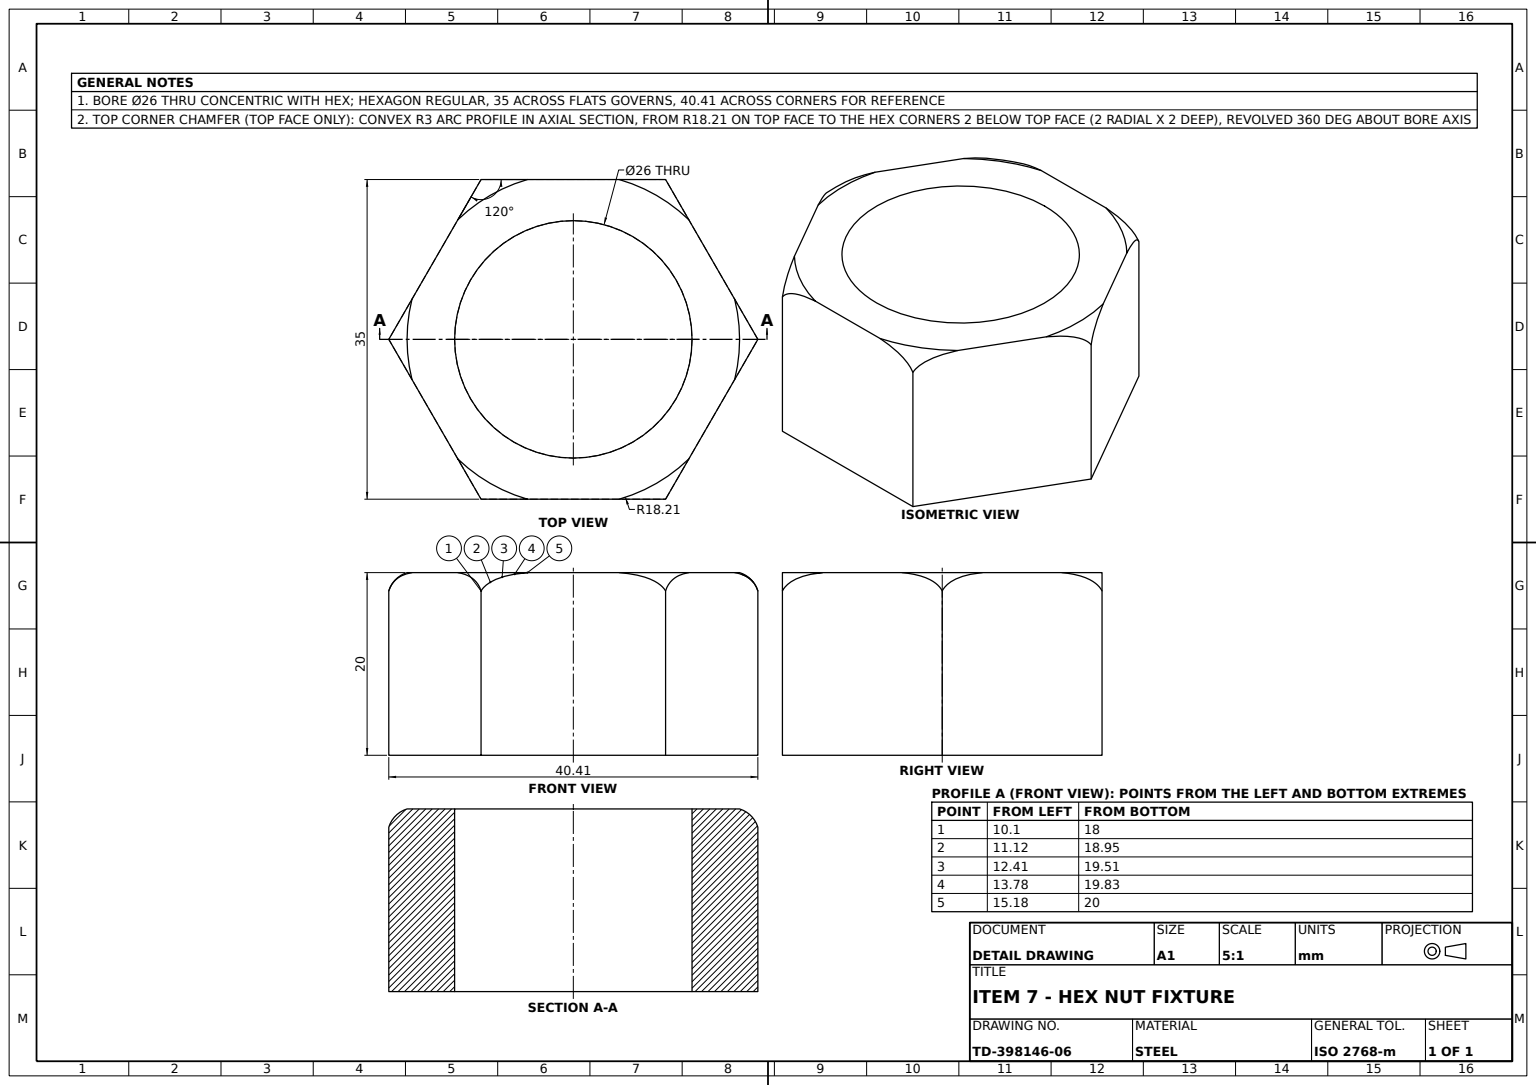
ISO-10303-21;
HEADER;
FILE_DESCRIPTION((''),'2;1');
FILE_NAME('','',(''),(''),'','','');
FILE_SCHEMA(('AUTOMOTIVE_DESIGN'));
ENDSEC;
DATA;
#1=APPLICATION_CONTEXT('');
#2=PRODUCT_CONTEXT('',#1,'mechanical');
#3=PRODUCT('','','',(#2));
#4=PRODUCT_DEFINITION_FORMATION('','',#3);
#5=PRODUCT_DEFINITION_CONTEXT('',#1,'design');
#6=PRODUCT_DEFINITION('','',#4,#5);
#7=PRODUCT_DEFINITION_SHAPE('','',#6);
#8=(LENGTH_UNIT()NAMED_UNIT(*)SI_UNIT(.MILLI.,.METRE.));
#9=(NAMED_UNIT(*)PLANE_ANGLE_UNIT()SI_UNIT($,.RADIAN.));
#10=(NAMED_UNIT(*)SI_UNIT($,.STERADIAN.)SOLID_ANGLE_UNIT());
#11=UNCERTAINTY_MEASURE_WITH_UNIT(LENGTH_MEASURE(1.E-05),#8,'distance_accuracy_value','');
#12=(GEOMETRIC_REPRESENTATION_CONTEXT(3)GLOBAL_UNCERTAINTY_ASSIGNED_CONTEXT((#11))GLOBAL_UNIT_ASSIGNED_CONTEXT((#8,#9,#10))REPRESENTATION_CONTEXT('',''));
#13=CARTESIAN_POINT('',(-10.10363,8.,17.5));
#14=VERTEX_POINT('',#13);
#15=CARTESIAN_POINT('',(-12.642762,10.,13.102094));
#16=VERTEX_POINT('',#15);
#17=CARTESIAN_POINT('',(-10.165722,8.204696,17.392454));
#18=CARTESIAN_POINT('',(-10.243014,8.380727,17.258579));
#19=CARTESIAN_POINT('',(-10.416921,8.69635,16.957363));
#20=CARTESIAN_POINT('',(-10.51443,8.835748,16.788473));
#21=CARTESIAN_POINT('',(-10.715898,9.077372,16.43952));
#22=CARTESIAN_POINT('',(-10.820898,9.181438,16.257655));
#23=CARTESIAN_POINT('',(-11.03705,9.365421,15.883269));
#24=CARTESIAN_POINT('',(-11.148709,9.445473,15.68987));
#25=CARTESIAN_POINT('',(-11.485835,9.654439,15.105951));
#26=CARTESIAN_POINT('',(-11.714336,9.754069,14.710176));
#27=CARTESIAN_POINT('',(-12.175668,9.907509,13.911124));
#28=CARTESIAN_POINT('',(-12.408551,9.960782,13.507759));
#29=B_SPLINE_CURVE_WITH_KNOTS('',3,(#13,#17,#18,#19,#20,#21,#22,#23,#24,#25,#26,#27,#28,#15),.UNSPECIFIED.,.F.,.F.,(4,2,2,2,2,2,4),(0.000000229,0.000702604,0.001404979,0.002107355,0.00280973,0.004214481,0.005619231),.UNSPECIFIED.);
#30=EDGE_CURVE('',#14,#16,#29,.T.);
#31=ORIENTED_EDGE('',*,*,#30,.F.);
#32=CARTESIAN_POINT('',(-5.025365,10.,17.5));
#33=VERTEX_POINT('',#32);
#34=CARTESIAN_POINT('',(-5.492104,9.960923,17.5));
#35=CARTESIAN_POINT('',(-5.960143,9.907453,17.5));
#36=CARTESIAN_POINT('',(-6.884053,9.753721,17.5));
#37=CARTESIAN_POINT('',(-7.33942,9.654067,17.5));
#38=CARTESIAN_POINT('',(-8.006087,9.447914,17.5));
#39=CARTESIAN_POINT('',(-8.225551,9.369653,17.5));
#40=CARTESIAN_POINT('',(-8.65696,9.187123,17.5));
#41=CARTESIAN_POINT('',(-8.870751,9.081899,17.5));
#42=CARTESIAN_POINT('',(-9.277733,8.838784,17.5));
#43=CARTESIAN_POINT('',(-9.470105,8.701958,17.5));
#44=CARTESIAN_POINT('',(-9.822347,8.383681,17.5));
#45=CARTESIAN_POINT('',(-9.980357,8.203194,17.5));
#46=B_SPLINE_CURVE_WITH_KNOTS('',3,(#32,#34,#35,#36,#37,#38,#39,#40,#41,#42,#43,#44,#45,#13),.UNSPECIFIED.,.F.,.F.,(4,2,2,2,2,2,4),(0.00502645,0.006430133,0.007833817,0.008535659,0.009237501,0.009939343,0.010641184),.UNSPECIFIED.);
#47=EDGE_CURVE('',#33,#14,#46,.T.);
#48=ORIENTED_EDGE('',*,*,#47,.F.);
#49=CARTESIAN_POINT('',(0.,10.,0.));
#50=DIRECTION('',(0.,-1.,0.));
#51=DIRECTION('',(0.,0.,-1.));
#52=AXIS2_PLACEMENT_3D('',#49,#50,#51);
#53=CIRCLE('',#52,18.207259);
#54=EDGE_CURVE('',#33,#16,#53,.T.);
#55=ORIENTED_EDGE('',*,*,#54,.T.);
#56=EDGE_LOOP('',(#31,#48,#55));
#57=FACE_OUTER_BOUND('',#56,.T.);
#58=CARTESIAN_POINT('',(0.,7.129171,0.));
#59=AXIS2_PLACEMENT_3D('',#58,#50,#51);
#60=TOROIDAL_SURFACE('',#59,17.336431,3.);
#61=ADVANCED_FACE('',(#57),#60,.T.);
#62=CARTESIAN_POINT('',(-10.10363,-10.,17.5));
#63=VERTEX_POINT('',#62);
#64=CARTESIAN_POINT('',(-10.10363,10.,17.5));
#65=VECTOR('',#50,1000.);
#66=LINE('',#64,#65);
#67=EDGE_CURVE('',#14,#63,#66,.T.);
#68=ORIENTED_EDGE('',*,*,#67,.F.);
#69=ORIENTED_EDGE('',*,*,#30,.T.);
#70=CARTESIAN_POINT('',(-17.668127,10.,4.397906));
#71=VERTEX_POINT('',#70);
#72=CARTESIAN_POINT('',(-20.207259,10.,0.));
#73=DIRECTION('',(0.5,0.,0.866025404));
#74=VECTOR('',#73,1000.);
#75=LINE('',#72,#74);
#76=EDGE_CURVE('',#71,#16,#75,.T.);
#77=ORIENTED_EDGE('',*,*,#76,.F.);
#78=CARTESIAN_POINT('',(-20.207259,8.,0.));
#79=VERTEX_POINT('',#78);
#80=CARTESIAN_POINT('',(-17.902082,9.960825,3.992684));
#81=CARTESIAN_POINT('',(-18.134693,9.907626,3.58979));
#82=CARTESIAN_POINT('',(-18.595438,9.754498,2.791757));
#83=CARTESIAN_POINT('',(-18.823622,9.655098,2.396531));
#84=CARTESIAN_POINT('',(-19.160225,9.446798,1.813516));
#85=CARTESIAN_POINT('',(-19.271845,9.366951,1.620186));
#86=CARTESIAN_POINT('',(-19.488371,9.182983,1.245151));
#87=CARTESIAN_POINT('',(-19.593676,9.078818,1.062757));
#88=CARTESIAN_POINT('',(-19.796013,8.836412,0.7123));
#89=CARTESIAN_POINT('',(-19.892647,8.698371,0.544925));
#90=CARTESIAN_POINT('',(-20.066575,8.383458,0.243673));
#91=CARTESIAN_POINT('',(-20.145542,8.203461,0.106897));
#92=B_SPLINE_CURVE_WITH_KNOTS('',3,(#70,#80,#81,#82,#83,#84,#85,#86,#87,#88,#89,#90,#91,#78),.UNSPECIFIED.,.F.,.F.,(4,2,2,2,2,2,4),(0.000002385,0.001403147,0.002803908,0.003504289,0.004204669,0.00490505,0.005605431),.UNSPECIFIED.);
#93=EDGE_CURVE('',#71,#79,#92,.T.);
#94=ORIENTED_EDGE('',*,*,#93,.T.);
#95=CARTESIAN_POINT('',(-20.207259,-10.,0.));
#96=VERTEX_POINT('',#95);
#97=LINE('',#72,#65);
#98=EDGE_CURVE('',#79,#96,#97,.T.);
#99=ORIENTED_EDGE('',*,*,#98,.T.);
#100=LINE('',#95,#74);
#101=EDGE_CURVE('',#96,#63,#100,.T.);
#102=ORIENTED_EDGE('',*,*,#101,.T.);
#103=EDGE_LOOP('',(#68,#69,#77,#94,#99,#102));
#104=FACE_OUTER_BOUND('',#103,.T.);
#105=DIRECTION('',(0.866025404,0.,-0.5));
#106=DIRECTION('',(-0.5,0.,-0.866025404));
#107=AXIS2_PLACEMENT_3D('',#72,#105,#106);
#108=PLANE('',#107);
#109=ADVANCED_FACE('',(#104),#108,.F.);
#110=CARTESIAN_POINT('',(10.10363,8.,-17.5));
#111=VERTEX_POINT('',#110);
#112=CARTESIAN_POINT('',(10.10363,-10.,-17.5));
#113=VERTEX_POINT('',#112);
#114=CARTESIAN_POINT('',(10.10363,10.,-17.5));
#115=LINE('',#114,#65);
#116=EDGE_CURVE('',#111,#113,#115,.T.);
#117=ORIENTED_EDGE('',*,*,#116,.T.);
#118=CARTESIAN_POINT('',(-10.10363,-10.,-17.5));
#119=VERTEX_POINT('',#118);
#120=DIRECTION('',(-1.,0.,0.));
#121=VECTOR('',#120,1000.);
#122=LINE('',#112,#121);
#123=EDGE_CURVE('',#113,#119,#122,.T.);
#124=ORIENTED_EDGE('',*,*,#123,.T.);
#125=CARTESIAN_POINT('',(-10.10363,8.,-17.5));
#126=VERTEX_POINT('',#125);
#127=CARTESIAN_POINT('',(-10.10363,10.,-17.5));
#128=LINE('',#127,#65);
#129=EDGE_CURVE('',#126,#119,#128,.T.);
#130=ORIENTED_EDGE('',*,*,#129,.F.);
#131=CARTESIAN_POINT('',(-5.025365,10.,-17.5));
#132=VERTEX_POINT('',#131);
#133=CARTESIAN_POINT('',(-9.98061,8.202777,-17.5));
#134=CARTESIAN_POINT('',(-9.825141,8.380727,-17.5));
#135=CARTESIAN_POINT('',(-9.473221,8.699564,-17.5));
#136=CARTESIAN_POINT('',(-9.282037,8.835729,-17.5));
#137=CARTESIAN_POINT('',(-8.87945,9.077171,-17.5));
#138=CARTESIAN_POINT('',(-8.666501,9.182682,-17.5));
#139=CARTESIAN_POINT('',(-8.233223,9.366796,-17.5));
#140=CARTESIAN_POINT('',(-8.012779,9.445661,-17.5));
#141=CARTESIAN_POINT('',(-7.343094,9.653291,-17.5));
#142=CARTESIAN_POINT('',(-6.885612,9.753482,-17.5));
#143=CARTESIAN_POINT('',(-5.957388,9.90789,-17.5));
#144=CARTESIAN_POINT('',(-5.491532,9.960971,-17.5));
#145=B_SPLINE_CURVE_WITH_KNOTS('',3,(#125,#133,#134,#135,#136,#137,#138,#139,#140,#141,#142,#143,#144,#131),.UNSPECIFIED.,.F.,.F.,(4,2,2,2,2,2,4),(0.035514707,0.036213744,0.036912782,0.037611819,0.038310856,0.039708931,0.041107005),.UNSPECIFIED.);
#146=EDGE_CURVE('',#126,#132,#145,.T.);
#147=ORIENTED_EDGE('',*,*,#146,.T.);
#148=CARTESIAN_POINT('',(5.025365,10.,-17.5));
#149=VERTEX_POINT('',#148);
#150=LINE('',#114,#121);
#151=EDGE_CURVE('',#149,#132,#150,.T.);
#152=ORIENTED_EDGE('',*,*,#151,.F.);
#153=CARTESIAN_POINT('',(5.492104,9.960923,-17.5));
#154=CARTESIAN_POINT('',(5.960143,9.907453,-17.5));
#155=CARTESIAN_POINT('',(6.884053,9.753721,-17.5));
#156=CARTESIAN_POINT('',(7.33942,9.654067,-17.5));
#157=CARTESIAN_POINT('',(8.006087,9.447914,-17.5));
#158=CARTESIAN_POINT('',(8.225551,9.369653,-17.5));
#159=CARTESIAN_POINT('',(8.65696,9.187123,-17.5));
#160=CARTESIAN_POINT('',(8.870751,9.081899,-17.5));
#161=CARTESIAN_POINT('',(9.277733,8.838784,-17.5));
#162=CARTESIAN_POINT('',(9.470105,8.701958,-17.5));
#163=CARTESIAN_POINT('',(9.822347,8.383681,-17.5));
#164=CARTESIAN_POINT('',(9.980357,8.203194,-17.5));
#165=B_SPLINE_CURVE_WITH_KNOTS('',3,(#148,#153,#154,#155,#156,#157,#158,#159,#160,#161,#162,#163,#164,#110),.UNSPECIFIED.,.F.,.F.,(4,2,2,2,2,2,4),(0.00502645,0.006430133,0.007833817,0.008535659,0.009237501,0.009939343,0.010641184),.UNSPECIFIED.);
#166=EDGE_CURVE('',#149,#111,#165,.T.);
#167=ORIENTED_EDGE('',*,*,#166,.T.);
#168=EDGE_LOOP('',(#117,#124,#130,#147,#152,#167));
#169=FACE_OUTER_BOUND('',#168,.T.);
#170=DIRECTION('',(0.,0.,1.));
#171=DIRECTION('',(1.,0.,0.));
#172=AXIS2_PLACEMENT_3D('',#114,#170,#171);
#173=PLANE('',#172);
#174=ADVANCED_FACE('',(#169),#173,.F.);
#175=CARTESIAN_POINT('',(10.10363,8.,17.5));
#176=VERTEX_POINT('',#175);
#177=CARTESIAN_POINT('',(5.025365,10.,17.5));
#178=VERTEX_POINT('',#177);
#179=CARTESIAN_POINT('',(9.98061,8.202777,17.5));
#180=CARTESIAN_POINT('',(9.825141,8.380727,17.5));
#181=CARTESIAN_POINT('',(9.473221,8.699564,17.5));
#182=CARTESIAN_POINT('',(9.282037,8.835729,17.5));
#183=CARTESIAN_POINT('',(8.87945,9.077171,17.5));
#184=CARTESIAN_POINT('',(8.666501,9.182682,17.5));
#185=CARTESIAN_POINT('',(8.233223,9.366796,17.5));
#186=CARTESIAN_POINT('',(8.012779,9.445661,17.5));
#187=CARTESIAN_POINT('',(7.343094,9.653291,17.5));
#188=CARTESIAN_POINT('',(6.885612,9.753482,17.5));
#189=CARTESIAN_POINT('',(5.957388,9.90789,17.5));
#190=CARTESIAN_POINT('',(5.491532,9.960971,17.5));
#191=B_SPLINE_CURVE_WITH_KNOTS('',3,(#175,#179,#180,#181,#182,#183,#184,#185,#186,#187,#188,#189,#190,#177),.UNSPECIFIED.,.F.,.F.,(4,2,2,2,2,2,4),(0.035514707,0.036213744,0.036912782,0.037611819,0.038310856,0.039708931,0.041107005),.UNSPECIFIED.);
#192=EDGE_CURVE('',#176,#178,#191,.T.);
#193=ORIENTED_EDGE('',*,*,#192,.F.);
#194=CARTESIAN_POINT('',(12.642762,10.,13.102094));
#195=VERTEX_POINT('',#194);
#196=CARTESIAN_POINT('',(12.408807,9.960825,13.507316));
#197=CARTESIAN_POINT('',(12.176196,9.907626,13.91021));
#198=CARTESIAN_POINT('',(11.715451,9.754498,14.708243));
#199=CARTESIAN_POINT('',(11.487267,9.655098,15.103469));
#200=CARTESIAN_POINT('',(11.150664,9.446798,15.686484));
#201=CARTESIAN_POINT('',(11.039045,9.366951,15.879814));
#202=CARTESIAN_POINT('',(10.822518,9.182983,16.254849));
#203=CARTESIAN_POINT('',(10.717213,9.078818,16.437243));
#204=CARTESIAN_POINT('',(10.514876,8.836412,16.7877));
#205=CARTESIAN_POINT('',(10.418243,8.698371,16.955075));
#206=CARTESIAN_POINT('',(10.244314,8.383458,17.256327));
#207=CARTESIAN_POINT('',(10.165347,8.203461,17.393103));
#208=B_SPLINE_CURVE_WITH_KNOTS('',3,(#194,#196,#197,#198,#199,#200,#201,#202,#203,#204,#205,#206,#207,#175),.UNSPECIFIED.,.F.,.F.,(4,2,2,2,2,2,4),(0.000002385,0.001403147,0.002803908,0.003504289,0.004204669,0.00490505,0.005605431),.UNSPECIFIED.);
#209=EDGE_CURVE('',#195,#176,#208,.T.);
#210=ORIENTED_EDGE('',*,*,#209,.F.);
#211=EDGE_CURVE('',#195,#178,#53,.T.);
#212=ORIENTED_EDGE('',*,*,#211,.T.);
#213=EDGE_LOOP('',(#193,#210,#212));
#214=FACE_OUTER_BOUND('',#213,.T.);
#215=ADVANCED_FACE('',(#214),#60,.T.);
#216=CARTESIAN_POINT('',(12.642762,10.,-13.102094));
#217=VERTEX_POINT('',#216);
#218=EDGE_CURVE('',#149,#217,#53,.T.);
#219=ORIENTED_EDGE('',*,*,#218,.T.);
#220=CARTESIAN_POINT('',(10.165722,8.204696,-17.392454));
#221=CARTESIAN_POINT('',(10.243014,8.380727,-17.258579));
#222=CARTESIAN_POINT('',(10.416921,8.69635,-16.957363));
#223=CARTESIAN_POINT('',(10.51443,8.835748,-16.788473));
#224=CARTESIAN_POINT('',(10.715898,9.077372,-16.43952));
#225=CARTESIAN_POINT('',(10.820898,9.181438,-16.257655));
#226=CARTESIAN_POINT('',(11.03705,9.365421,-15.883269));
#227=CARTESIAN_POINT('',(11.148709,9.445473,-15.68987));
#228=CARTESIAN_POINT('',(11.485835,9.654439,-15.105951));
#229=CARTESIAN_POINT('',(11.714336,9.754069,-14.710176));
#230=CARTESIAN_POINT('',(12.175668,9.907509,-13.911124));
#231=CARTESIAN_POINT('',(12.408551,9.960782,-13.507759));
#232=B_SPLINE_CURVE_WITH_KNOTS('',3,(#110,#220,#221,#222,#223,#224,#225,#226,#227,#228,#229,#230,#231,#216),.UNSPECIFIED.,.F.,.F.,(4,2,2,2,2,2,4),(0.000000229,0.000702604,0.001404979,0.002107355,0.00280973,0.004214481,0.005619231),.UNSPECIFIED.);
#233=EDGE_CURVE('',#111,#217,#232,.T.);
#234=ORIENTED_EDGE('',*,*,#233,.F.);
#235=ORIENTED_EDGE('',*,*,#166,.F.);
#236=EDGE_LOOP('',(#219,#234,#235));
#237=FACE_OUTER_BOUND('',#236,.T.);
#238=ADVANCED_FACE('',(#237),#60,.T.);
#239=DIRECTION('',(-0.5,0.,0.866025404));
#240=VECTOR('',#239,1000.);
#241=LINE('',#118,#240);
#242=EDGE_CURVE('',#119,#96,#241,.T.);
#243=ORIENTED_EDGE('',*,*,#242,.T.);
#244=ORIENTED_EDGE('',*,*,#98,.F.);
#245=CARTESIAN_POINT('',(-17.668127,10.,-4.397906));
#246=VERTEX_POINT('',#245);
#247=CARTESIAN_POINT('',(-20.145167,8.204696,-0.107546));
#248=CARTESIAN_POINT('',(-20.067875,8.380727,-0.241421));
#249=CARTESIAN_POINT('',(-19.893968,8.69635,-0.542637));
#250=CARTESIAN_POINT('',(-19.796459,8.835748,-0.711527));
#251=CARTESIAN_POINT('',(-19.594991,9.077372,-1.06048));
#252=CARTESIAN_POINT('',(-19.489991,9.181438,-1.242345));
#253=CARTESIAN_POINT('',(-19.273839,9.365421,-1.616731));
#254=CARTESIAN_POINT('',(-19.16218,9.445473,-1.81013));
#255=CARTESIAN_POINT('',(-18.825055,9.654439,-2.394049));
#256=CARTESIAN_POINT('',(-18.596554,9.754069,-2.789824));
#257=CARTESIAN_POINT('',(-18.135221,9.907509,-3.588876));
#258=CARTESIAN_POINT('',(-17.902338,9.960782,-3.992241));
#259=B_SPLINE_CURVE_WITH_KNOTS('',3,(#78,#247,#248,#249,#250,#251,#252,#253,#254,#255,#256,#257,#258,#245),.UNSPECIFIED.,.F.,.F.,(4,2,2,2,2,2,4),(0.000000229,0.000702604,0.001404979,0.002107355,0.00280973,0.004214481,0.005619231),.UNSPECIFIED.);
#260=EDGE_CURVE('',#79,#246,#259,.T.);
#261=ORIENTED_EDGE('',*,*,#260,.T.);
#262=CARTESIAN_POINT('',(-12.642762,10.,-13.102094));
#263=VERTEX_POINT('',#262);
#264=LINE('',#127,#240);
#265=EDGE_CURVE('',#263,#246,#264,.T.);
#266=ORIENTED_EDGE('',*,*,#265,.F.);
#267=CARTESIAN_POINT('',(-12.408807,9.960825,-13.507316));
#268=CARTESIAN_POINT('',(-12.176196,9.907626,-13.91021));
#269=CARTESIAN_POINT('',(-11.715451,9.754498,-14.708243));
#270=CARTESIAN_POINT('',(-11.487267,9.655098,-15.103469));
#271=CARTESIAN_POINT('',(-11.150664,9.446798,-15.686484));
#272=CARTESIAN_POINT('',(-11.039045,9.366951,-15.879814));
#273=CARTESIAN_POINT('',(-10.822518,9.182983,-16.254849));
#274=CARTESIAN_POINT('',(-10.717213,9.078818,-16.437243));
#275=CARTESIAN_POINT('',(-10.514876,8.836412,-16.7877));
#276=CARTESIAN_POINT('',(-10.418243,8.698371,-16.955075));
#277=CARTESIAN_POINT('',(-10.244314,8.383458,-17.256327));
#278=CARTESIAN_POINT('',(-10.165347,8.203461,-17.393103));
#279=B_SPLINE_CURVE_WITH_KNOTS('',3,(#262,#267,#268,#269,#270,#271,#272,#273,#274,#275,#276,#277,#278,#125),.UNSPECIFIED.,.F.,.F.,(4,2,2,2,2,2,4),(0.000002385,0.001403147,0.002803908,0.003504289,0.004204669,0.00490505,0.005605431),.UNSPECIFIED.);
#280=EDGE_CURVE('',#263,#126,#279,.T.);
#281=ORIENTED_EDGE('',*,*,#280,.T.);
#282=ORIENTED_EDGE('',*,*,#129,.T.);
#283=EDGE_LOOP('',(#243,#244,#261,#266,#281,#282));
#284=FACE_OUTER_BOUND('',#283,.T.);
#285=DIRECTION('',(0.866025404,0.,0.5));
#286=DIRECTION('',(0.5,0.,-0.866025404));
#287=AXIS2_PLACEMENT_3D('',#127,#285,#286);
#288=PLANE('',#287);
#289=ADVANCED_FACE('',(#284),#288,.F.);
#290=EDGE_CURVE('',#71,#246,#53,.T.);
#291=ORIENTED_EDGE('',*,*,#290,.T.);
#292=ORIENTED_EDGE('',*,*,#260,.F.);
#293=ORIENTED_EDGE('',*,*,#93,.F.);
#294=EDGE_LOOP('',(#291,#292,#293));
#295=FACE_OUTER_BOUND('',#294,.T.);
#296=ADVANCED_FACE('',(#295),#60,.T.);
#297=CARTESIAN_POINT('',(0.,10.,-13.));
#298=VERTEX_POINT('',#297);
#299=CARTESIAN_POINT('',(0.,-10.,-13.));
#300=VERTEX_POINT('',#299);
#301=LINE('',#297,#65);
#302=EDGE_CURVE('',#298,#300,#301,.T.);
#303=ORIENTED_EDGE('',*,*,#302,.T.);
#304=CARTESIAN_POINT('',(0.,-10.,13.));
#305=VERTEX_POINT('',#304);
#306=CARTESIAN_POINT('',(0.,-10.,0.));
#307=DIRECTION('',(0.,1.,0.));
#308=AXIS2_PLACEMENT_3D('',#306,#307,#170);
#309=CIRCLE('',#308,13.);
#310=EDGE_CURVE('',#305,#300,#309,.T.);
#311=ORIENTED_EDGE('',*,*,#310,.F.);
#312=CARTESIAN_POINT('',(0.,10.,13.));
#313=VERTEX_POINT('',#312);
#314=LINE('',#312,#65);
#315=EDGE_CURVE('',#313,#305,#314,.T.);
#316=ORIENTED_EDGE('',*,*,#315,.F.);
#317=AXIS2_PLACEMENT_3D('',#49,#307,#170);
#318=CIRCLE('',#317,13.);
#319=EDGE_CURVE('',#313,#298,#318,.T.);
#320=ORIENTED_EDGE('',*,*,#319,.T.);
#321=EDGE_LOOP('',(#303,#311,#316,#320));
#322=FACE_OUTER_BOUND('',#321,.T.);
#323=CYLINDRICAL_SURFACE('',#52,13.);
#324=ADVANCED_FACE('',(#322),#323,.F.);
#325=CARTESIAN_POINT('',(17.668127,10.,-4.397906));
#326=VERTEX_POINT('',#325);
#327=CARTESIAN_POINT('',(20.207259,8.,0.));
#328=VERTEX_POINT('',#327);
#329=CARTESIAN_POINT('',(17.902082,9.960825,-3.992684));
#330=CARTESIAN_POINT('',(18.134693,9.907626,-3.58979));
#331=CARTESIAN_POINT('',(18.595438,9.754498,-2.791757));
#332=CARTESIAN_POINT('',(18.823622,9.655098,-2.396531));
#333=CARTESIAN_POINT('',(19.160225,9.446798,-1.813516));
#334=CARTESIAN_POINT('',(19.271845,9.366951,-1.620186));
#335=CARTESIAN_POINT('',(19.488371,9.182983,-1.245151));
#336=CARTESIAN_POINT('',(19.593676,9.078818,-1.062757));
#337=CARTESIAN_POINT('',(19.796013,8.836412,-0.7123));
#338=CARTESIAN_POINT('',(19.892647,8.698371,-0.544925));
#339=CARTESIAN_POINT('',(20.066575,8.383458,-0.243673));
#340=CARTESIAN_POINT('',(20.145542,8.203461,-0.106897));
#341=B_SPLINE_CURVE_WITH_KNOTS('',3,(#325,#329,#330,#331,#332,#333,#334,#335,#336,#337,#338,#339,#340,#327),.UNSPECIFIED.,.F.,.F.,(4,2,2,2,2,2,4),(0.000002385,0.001403147,0.002803908,0.003504289,0.004204669,0.00490505,0.005605431),.UNSPECIFIED.);
#342=EDGE_CURVE('',#326,#328,#341,.T.);
#343=ORIENTED_EDGE('',*,*,#342,.F.);
#344=CARTESIAN_POINT('',(17.668127,10.,4.397906));
#345=VERTEX_POINT('',#344);
#346=EDGE_CURVE('',#326,#345,#53,.T.);
#347=ORIENTED_EDGE('',*,*,#346,.T.);
#348=CARTESIAN_POINT('',(20.145167,8.204696,0.107546));
#349=CARTESIAN_POINT('',(20.067875,8.380727,0.241421));
#350=CARTESIAN_POINT('',(19.893968,8.69635,0.542637));
#351=CARTESIAN_POINT('',(19.796459,8.835748,0.711527));
#352=CARTESIAN_POINT('',(19.594991,9.077372,1.06048));
#353=CARTESIAN_POINT('',(19.489991,9.181438,1.242345));
#354=CARTESIAN_POINT('',(19.273839,9.365421,1.616731));
#355=CARTESIAN_POINT('',(19.16218,9.445473,1.81013));
#356=CARTESIAN_POINT('',(18.825055,9.654439,2.394049));
#357=CARTESIAN_POINT('',(18.596554,9.754069,2.789824));
#358=CARTESIAN_POINT('',(18.135221,9.907509,3.588876));
#359=CARTESIAN_POINT('',(17.902338,9.960782,3.992241));
#360=B_SPLINE_CURVE_WITH_KNOTS('',3,(#327,#348,#349,#350,#351,#352,#353,#354,#355,#356,#357,#358,#359,#344),.UNSPECIFIED.,.F.,.F.,(4,2,2,2,2,2,4),(0.000000229,0.000702604,0.001404979,0.002107355,0.00280973,0.004214481,0.005619231),.UNSPECIFIED.);
#361=EDGE_CURVE('',#328,#345,#360,.T.);
#362=ORIENTED_EDGE('',*,*,#361,.F.);
#363=EDGE_LOOP('',(#343,#347,#362));
#364=FACE_OUTER_BOUND('',#363,.T.);
#365=ADVANCED_FACE('',(#364),#60,.T.);
#366=ORIENTED_EDGE('',*,*,#233,.T.);
#367=CARTESIAN_POINT('',(20.207259,10.,0.));
#368=VECTOR('',#106,1000.);
#369=LINE('',#367,#368);
#370=EDGE_CURVE('',#326,#217,#369,.T.);
#371=ORIENTED_EDGE('',*,*,#370,.F.);
#372=ORIENTED_EDGE('',*,*,#342,.T.);
#373=CARTESIAN_POINT('',(20.207259,-10.,0.));
#374=VERTEX_POINT('',#373);
#375=LINE('',#367,#65);
#376=EDGE_CURVE('',#328,#374,#375,.T.);
#377=ORIENTED_EDGE('',*,*,#376,.T.);
#378=LINE('',#373,#368);
#379=EDGE_CURVE('',#374,#113,#378,.T.);
#380=ORIENTED_EDGE('',*,*,#379,.T.);
#381=ORIENTED_EDGE('',*,*,#116,.F.);
#382=EDGE_LOOP('',(#366,#371,#372,#377,#380,#381));
#383=FACE_OUTER_BOUND('',#382,.T.);
#384=DIRECTION('',(-0.866025404,0.,0.5));
#385=AXIS2_PLACEMENT_3D('',#367,#384,#73);
#386=PLANE('',#385);
#387=ADVANCED_FACE('',(#383),#386,.F.);
#388=ORIENTED_EDGE('',*,*,#146,.F.);
#389=ORIENTED_EDGE('',*,*,#280,.F.);
#390=EDGE_CURVE('',#263,#132,#53,.T.);
#391=ORIENTED_EDGE('',*,*,#390,.T.);
#392=EDGE_LOOP('',(#388,#389,#391));
#393=FACE_OUTER_BOUND('',#392,.T.);
#394=ADVANCED_FACE('',(#393),#60,.T.);
#395=ORIENTED_EDGE('',*,*,#319,.F.);
#396=EDGE_CURVE('',#298,#313,#318,.T.);
#397=ORIENTED_EDGE('',*,*,#396,.F.);
#398=EDGE_LOOP('',(#395,#397));
#399=FACE_BOUND('',#398,.T.);
#400=ORIENTED_EDGE('',*,*,#265,.T.);
#401=ORIENTED_EDGE('',*,*,#290,.F.);
#402=ORIENTED_EDGE('',*,*,#76,.T.);
#403=ORIENTED_EDGE('',*,*,#54,.F.);
#404=VECTOR('',#171,1000.);
#405=LINE('',#64,#404);
#406=EDGE_CURVE('',#33,#178,#405,.T.);
#407=ORIENTED_EDGE('',*,*,#406,.T.);
#408=ORIENTED_EDGE('',*,*,#211,.F.);
#409=CARTESIAN_POINT('',(10.10363,10.,17.5));
#410=VECTOR('',#286,1000.);
#411=LINE('',#409,#410);
#412=EDGE_CURVE('',#195,#345,#411,.T.);
#413=ORIENTED_EDGE('',*,*,#412,.T.);
#414=ORIENTED_EDGE('',*,*,#346,.F.);
#415=ORIENTED_EDGE('',*,*,#370,.T.);
#416=ORIENTED_EDGE('',*,*,#218,.F.);
#417=ORIENTED_EDGE('',*,*,#151,.T.);
#418=ORIENTED_EDGE('',*,*,#390,.F.);
#419=EDGE_LOOP('',(#400,#401,#402,#403,#407,#408,#413,#414,#415,#416,#417,#418));
#420=FACE_OUTER_BOUND('',#419,.T.);
#421=PLANE('',#317);
#422=ADVANCED_FACE('',(#399,#420),#421,.T.);
#423=ORIENTED_EDGE('',*,*,#376,.F.);
#424=ORIENTED_EDGE('',*,*,#361,.T.);
#425=ORIENTED_EDGE('',*,*,#412,.F.);
#426=ORIENTED_EDGE('',*,*,#209,.T.);
#427=CARTESIAN_POINT('',(10.10363,-10.,17.5));
#428=VERTEX_POINT('',#427);
#429=LINE('',#409,#65);
#430=EDGE_CURVE('',#176,#428,#429,.T.);
#431=ORIENTED_EDGE('',*,*,#430,.T.);
#432=LINE('',#427,#410);
#433=EDGE_CURVE('',#428,#374,#432,.T.);
#434=ORIENTED_EDGE('',*,*,#433,.T.);
#435=EDGE_LOOP('',(#423,#424,#425,#426,#431,#434));
#436=FACE_OUTER_BOUND('',#435,.T.);
#437=DIRECTION('',(-0.866025404,0.,-0.5));
#438=AXIS2_PLACEMENT_3D('',#409,#437,#239);
#439=PLANE('',#438);
#440=ADVANCED_FACE('',(#436),#439,.F.);
#441=ORIENTED_EDGE('',*,*,#242,.F.);
#442=ORIENTED_EDGE('',*,*,#123,.F.);
#443=ORIENTED_EDGE('',*,*,#379,.F.);
#444=ORIENTED_EDGE('',*,*,#433,.F.);
#445=LINE('',#62,#404);
#446=EDGE_CURVE('',#63,#428,#445,.T.);
#447=ORIENTED_EDGE('',*,*,#446,.F.);
#448=ORIENTED_EDGE('',*,*,#101,.F.);
#449=EDGE_LOOP('',(#441,#442,#443,#444,#447,#448));
#450=FACE_OUTER_BOUND('',#449,.T.);
#451=ORIENTED_EDGE('',*,*,#310,.T.);
#452=EDGE_CURVE('',#300,#305,#309,.T.);
#453=ORIENTED_EDGE('',*,*,#452,.T.);
#454=EDGE_LOOP('',(#451,#453));
#455=FACE_BOUND('',#454,.T.);
#456=PLANE('',#308);
#457=ADVANCED_FACE('',(#450,#455),#456,.F.);
#458=ORIENTED_EDGE('',*,*,#406,.F.);
#459=ORIENTED_EDGE('',*,*,#47,.T.);
#460=ORIENTED_EDGE('',*,*,#67,.T.);
#461=ORIENTED_EDGE('',*,*,#446,.T.);
#462=ORIENTED_EDGE('',*,*,#430,.F.);
#463=ORIENTED_EDGE('',*,*,#192,.T.);
#464=EDGE_LOOP('',(#458,#459,#460,#461,#462,#463));
#465=FACE_OUTER_BOUND('',#464,.T.);
#466=AXIS2_PLACEMENT_3D('',#64,#51,#120);
#467=PLANE('',#466);
#468=ADVANCED_FACE('',(#465),#467,.F.);
#469=ORIENTED_EDGE('',*,*,#452,.F.);
#470=ORIENTED_EDGE('',*,*,#302,.F.);
#471=ORIENTED_EDGE('',*,*,#396,.T.);
#472=ORIENTED_EDGE('',*,*,#315,.T.);
#473=EDGE_LOOP('',(#469,#470,#471,#472));
#474=FACE_OUTER_BOUND('',#473,.T.);
#475=ADVANCED_FACE('',(#474),#323,.F.);
#476=CLOSED_SHELL('',(#61,#109,#174,#215,#238,#289,#296,#324,#365,#387,#394,#422,#440,#457,#468,#475));
#477=MANIFOLD_SOLID_BREP('',#476);
#478=ADVANCED_BREP_SHAPE_REPRESENTATION('',(#477),#12);
#479=SHAPE_DEFINITION_REPRESENTATION(#7,#478);
ENDSEC;
END-ISO-10303-21;
